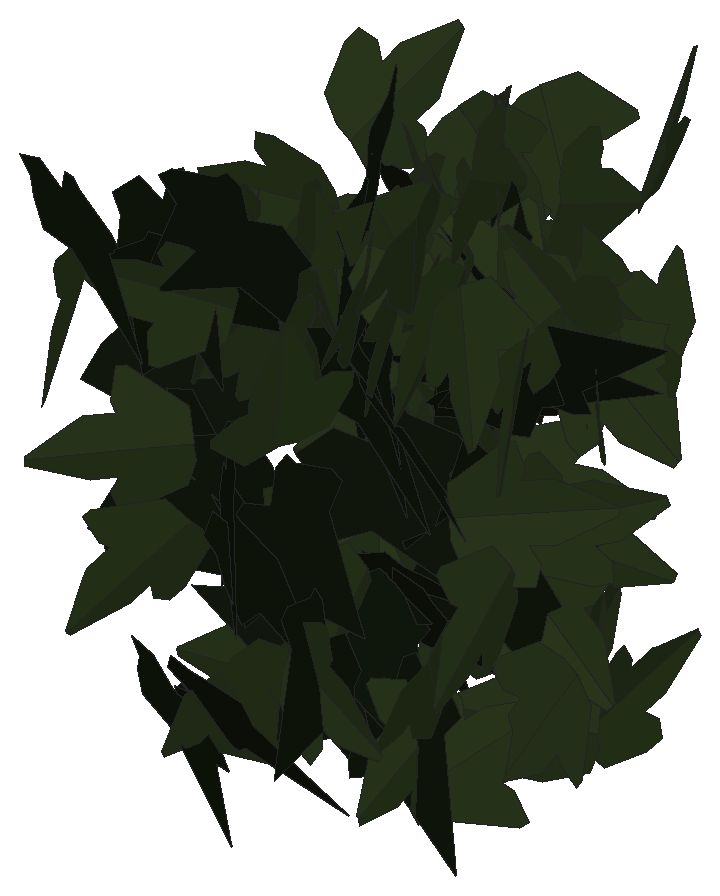
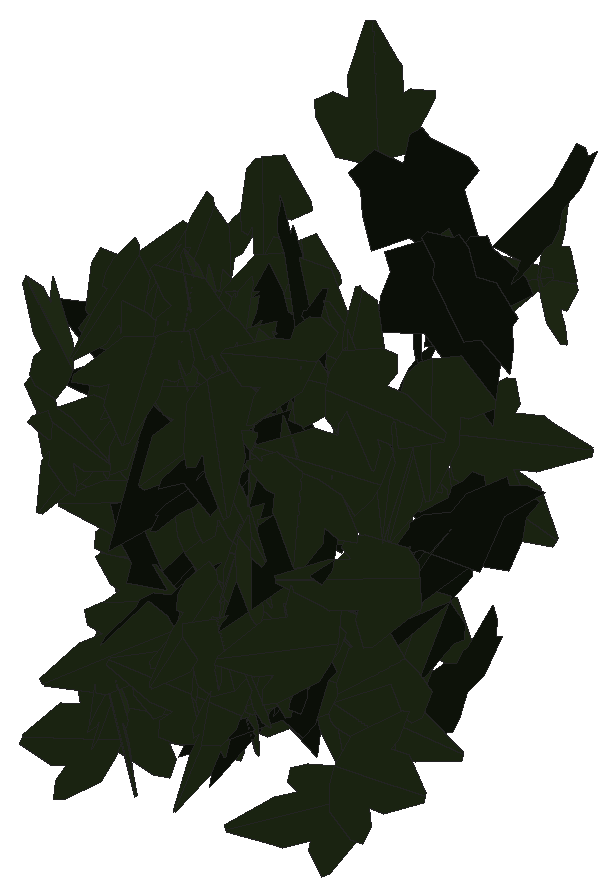
# SketchUp Ruby script. Lengths in inches.
U = 1.inch
M = Sketchup.active_model
def pt(a) = Geom::Point3d.new(a.map { |v| v * U })
def face(e, loops, mat)
  f = e.add_face(loops[0].map { |a| pt(a) })
  loops[1..].each { |l| e.add_face(l.map { |a| pt(a) }).erase! }
  f.material = f.back_material = mat if mat
  f
end
# faces: each face lists its corners as indices into pts; further lists are holes
def faces(e, pts, list, mat = nil) = list.each { |f| face(e, (f[0].is_a?(Array) ? f : [f]).map { |l| l.map { |i| pts[i] } }, mat) }
# xy, xz, yz: faces in a plane at the given z, y or x. An outline is a flat list of corners, or four numbers for a rectangle; further outlines are holes
def ring(l) = l.size == 4 ? [[l[0], l[1]], [l[2], l[1]], [l[2], l[3]], [l[0], l[3]]] : l.each_slice(2).to_a
def flat(e, list, mat, &to3) = list.each { |f| face(e, (f[0].is_a?(Array) ? f : [f]).map { |l| ring(l).map { |u, v| to3.(u, v) } }, mat) }
def xy(e, z, list, mat = nil) = flat(e, list, mat) { |x, y| [x, y, z] }
def xz(e, y, list, mat = nil) = flat(e, list, mat) { |x, z| [x, y, z] }
def yz(e, x, list, mat = nil) = flat(e, list, mat) { |y, z| [x, y, z] }
def lines(e, pts, list) = list.each { |a, b| e.add_line(pt(pts[a]), pt(pts[b])) }
# prism: a flat outline (further loops are holes) pulled along v
def prism(e, loops, v, mat = nil)
  f = face(e, loops, mat); d = Geom::Vector3d.new(v.map { |x| x * U })
  f.pushpull(f.normal.samedirection?(d) ? d.length : -d.length)
end
def box(e, o, s, mat = nil) = prism(e, [[o, [o[0] + s[0], o[1], o[2]], [o[0] + s[0], o[1] + s[1], o[2]], [o[0], o[1] + s[1], o[2]]]], [0, 0, s[2]], mat)
def at(x, y, z, deg = 0) = Geom::Transformation.translation(pt([x, y, z])) * Geom::Transformation.rotation(ORIGIN, Z_AXIS, deg.degrees)
def axes(o, x, y, z) = Geom::Transformation.new([*x, 0, *y, 0, *z, 0, *pt(o).to_a, 1])
def part(name) = M.definitions.add(name)
# library, detail: a bought-in or finely detailed component or shape, given as its bounding box
def library(name, o, s) = part(name).tap { |d| box(d.entities, o, s) }
def detail(e, o, s) = box(e.add_group.entities, o, s)
def put(e, d, t, mat = nil) = e.add_instance(d, t).tap { |i| i.material = mat if mat }
def group(e, t, mat = nil) = e.add_group.tap { |g| g.transformation = t; g.material = mat if mat }.entities
root = M.entities
M.materials.add("efeu1").color = [18, 25, 13]
M.materials.add("efeu2").color = [43, 57, 29]
c1 = part("ivyleaf_10")
p = [[0,0.5,-0.03],[-0.0625,2.02,-0.43],[-0.19,2.01,-0.46],[-0.54,1.05,-0.29],[-0.52,0.625,-0.18],[-0.83,0.76,-0.28],
  [-1.16,0.64,-0.33],[-1.15,0.33,-0.24],[-0.77,-0.39,0.02],[-0.3,-0.51,0.16],[0.04,-0.48,0.23],[-0.02,2.01,-0.4375],
  [-0.06,2.01,-0.43],[0.04,-0.49,0.23],[0.67,-0.49,0.14],[1.38,0.36,-0.2],[1.375,0.51,-0.24],[0.81,0.65,-0.19],
  [0.62,0.59,-0.15],[0.6,1.09,-0.28],[0.5,1.23,-0.31]]
faces(c1.entities,p,[[0,1,2,3,4,5,6,7,8,9,10],[11,12,0,13,14,15,16,17,18,19,20]],"efeu2")
c2 = part("ivyleaf_9")
p = [[1.54,2.16,1.25],[1.36,2.04,1.19],[-0.21,0.99,0.68],[-0.71,1.11,0.82],[-0.85,0.86,0.67],[-0.8,0.17,0.21],
  [-0.9,-0.01,0.1],[-0.67,-0.16,-0.02],[-0.08,-0.08,-0.05],[-0.03,-0.6,-0.4],[0.65,-0.88,-0.66],[0.83,-0.6,-0.49],
  [1.29,-0.42,-0.43],[1.8125,-0.07,-0.26],[1.21,0.44,0.15]]
faces(c2.entities,p,[[0,1,2,3,4,5,6,7,8,9,10,11,12,13,14]],"efeu1")
put(root,c1,axes([15.76,224.72,205.29],[-0.06283,0.04906,0.49361],[-0.33114,0.3663,-0.07855],[-0.36932,-0.33678,-0.01354]))
put(root,c2,axes([15.47,224.3125,204.75],[-0.14625,-0.47747,-0.02524],[0.00758,0.02408,-0.49936],[0.47807,-0.14645,0.00019]))
put(root,c1,axes([15.59,225.57,202.5625],[-0.03739,-0.25538,0.42823],[0.05297,-0.42904,-0.25124],[0.49578,0.02658,0.05913]))
put(root,c1,axes([15.72,224.28,205.94],[-0.08357,-0.48272,-0.09997],[0.02692,0.09678,-0.48981],[0.49223,-0.08725,0.00982]))
put(root,c1,axes([16.13,224.9375,206],[0.05956,0.01203,-0.49629],[-0.48805,0.09294,-0.05632],[0.0909,0.49114,0.02281]))
put(root,c1,axes([15.86,224.29,205.39],[0.0225,-0.33473,-0.37074],[-0.00859,0.37081,-0.3353],[0.49942,0.02146,0.01094]))
put(root,c1,axes([15.53,225.16,204.41],[0.00781,-0.06414,-0.49581],[0.46045,0.19407,-0.01786],[0.19473,-0.45631,0.0621]))
put(root,c1,axes([16.17,223.08,204.72],[-0.02892,-0.02669,0.49845],[-0.30325,-0.39565,-0.03878],[0.39649,-0.30455,0.0067]))
put(root,c1,axes([16.04,224.69,204.98],[-0.13643,-0.48097,-0.00753],[0.00223,0.00719,-0.49994],[0.48102,-0.13645,0.00019]))
put(root,c1,axes([15.82,222.48,206.24],[0.13321,-0.20511,0.4361],[0.26583,-0.34613,-0.24399],[0.40198,0.29686,0.01684]))
put(root,c2,axes([15.71,222.5,206.99],[0.29313,-0.39372,0.09519],[0.05753,-0.07585,-0.49085],[0.40096,0.29872,0.00083]))
put(root,c2,axes([15.79,224.27,204.2],[0.21036,-0.45026,0.05495],[0.02428,-0.04931,-0.49697],[0.45295,0.21175,0.00112]))
put(root,c2,axes([15.97,223.27,204.2],[0.06582,-0.16806,-0.46629],[-0.11073,0.4535,-0.17909],[0.48312,0.12684,0.02248]))
put(root,c1,axes([15.85,225.52,202.15],[-0.02924,-0.09795,-0.48944],[0.3953,0.29481,-0.08261],[0.30477,-0.39178,0.0602]))
put(root,c1,axes([16.5,224.26,202.28],[-0.01794,-0.00235,0.49967],[-0.47822,-0.14488,-0.01785],[0.14487,-0.47854,0.00295]))
put(root,c2,axes([15.97,223.39,206.58],[-0.18584,-0.06121,-0.46013],[0.43336,0.15472,-0.19561],[0.16633,-0.4715,-0.00445]))
put(root,c1,axes([16.07,225.72,205.41],[0.4797,0.0215,0.13937],[0.13869,0.0175,-0.48006],[-0.02552,0.49923,0.01083]))
put(root,c1,axes([16.15,225.53,203.68],[-0.02079,-0.10534,0.48833],[0.0401,0.48683,0.10672],[-0.49796,0.0436,-0.0118]))
put(root,c1,axes([16.08,225,205.23],[-0.08764,-0.22092,0.4399],[0.152,0.41284,0.23761],[-0.4682,0.17538,-0.00521]))
put(root,c1,axes([16.59,223.06,206.12],[-0.12984,0.02802,-0.48203],[-0.46825,-0.12909,0.11863],[-0.11781,0.48223,0.05977]))
put(root,c1,axes([15.91,224.65,203.18],[0.30613,0.07602,0.38795],[0.37679,0.09236,-0.31543],[-0.11962,0.48548,-0.00073]))
put(root,c1,axes([16.42,222.83,204.08],[-0.11373,-0.31356,0.37249],[-0.13234,-0.3482,-0.33353],[0.46856,-0.17445,-0.00379]))
put(root,c2,axes([16.47,223.09,206.39],[0.20451,0.29275,-0.34996],[-0.22048,-0.27235,-0.35667],[-0.39945,0.3002,0.01769]))
put(root,c2,axes([16.05,223.43,202.33],[0.22091,-0.3855,0.22932],[0.11019,-0.20115,-0.44429],[0.43481,0.24683,-0.00392]))
put(root,c1,axes([16.27,225.52,206.5625],[0.18062,0.15706,-0.43899],[0.18473,0.40814,0.22203],[0.42808,-0.24239,0.08941]))
put(root,c1,axes([16.04,224.67,202.46],[-0.06526,-0.015,0.4955],[0.49403,0.03926,0.06626],[-0.0409,0.49823,0.0097]))
put(root,c1,axes([16.51,224.59,205.26],[0.14733,-0.37725,-0.29321],[-0.0089,0.30462,-0.3964],[0.47772,0.12202,0.08304]))
put(root,c2,axes([16.39,225.22,204.9],[0.49076,0.00696,-0.09543],[-0.09554,0.00754,-0.49073],[-0.00539,0.49989,0.00873]))
put(root,c1,axes([16.92,225.35,204.16],[-0.09164,-0.10191,0.48085],[-0.35318,-0.32654,-0.13652],[0.34186,-0.36467,-0.01214]))
put(root,c1,axes([16.7,226.23,206.24],[-0.00117,-0.49927,-0.02693],[0.0006,0.02692,-0.49927],[0.5,-0.0012,0.00054]))
put(root,c1,axes([16.71,224.1,206.24],[0.08895,-0.35534,-0.34032],[-0.01174,0.34421,-0.36247],[0.49188,0.07247,0.05289]))
put(root,c1,axes([16.79,224.48,202.8],[-0.0375,-0.49823,0.01897],[-0.00181,-0.01889,-0.49964],[0.49859,-0.03754,-0.00038]))
put(root,c1,axes([16.74,223.22,202.75],[-0.17653,-0.40832,-0.22829],[0.11011,0.20088,-0.44443],[0.45466,-0.20718,0.01899]))
put(root,c1,axes([16.52,224.52,206],[-0.16226,0.12848,-0.45515],[0.28535,-0.35715,-0.20254],[-0.37716,-0.32548,0.04257]))
put(root,c1,axes([16.87,225.11,205.64],[0.30259,-0.35449,-0.18104],[-0.11969,0.13585,-0.46607],[0.37962,0.3254,-0.00265]))
put(root,c2,axes([17,224.43,202.51],[-0.11716,-0.45808,-0.16259],[-0.04226,-0.15701,0.47282],[-0.48424,0.12453,-0.00193]))
put(root,c1,axes([16.73,225.0625,203.01],[-0.02487,0.07316,0.49399],[0.14637,-0.47182,0.07724],[0.47745,0.14845,0.00205]))
put(root,c1,axes([16.61,225.01,203.17],[0.17938,0.15112,-0.44157],[0.34288,0.27827,0.23452],[0.31663,-0.38695,-0.0038]))
put(root,c2,axes([17.15,222.89,207.09],[0.08905,0.13143,-0.47413],[-0.37355,-0.29553,-0.15208],[-0.32021,0.3813,0.04556]))
put(root,c1,axes([16.62,224.8125,202.86],[0.17627,0.12899,-0.44977],[0.35177,0.28038,0.21827],[0.30852,-0.39338,0.0081]))
put(root,c1,axes([16.94,225.29,205.92],[0.17758,-0.37267,-0.28211],[-0.04572,0.28649,-0.40723],[0.46516,0.17043,0.06767]))
put(root,c1,axes([16.85,225.46,204.37],[0.12139,-0.38738,0.29189],[0.10185,-0.27383,-0.40576],[0.47423,0.15797,0.01243]))
put(root,c2,axes([17.23,224.46,207.01],[-0.0952,0.02704,-0.49011],[-0.45859,0.17312,0.09862],[0.17503,0.46829,-0.00816]))
put(root,c1,axes([16.93,225.47,206.18],[0.10483,-0.39249,0.29148],[0.06972,-0.28306,-0.40622],[0.48389,0.12581,-0.00462]))
put(root,c1,axes([16.99,225.75,203.59],[0.35154,0.3454,-0.08437],[-0.06164,-0.05764,-0.49283],[-0.35017,0.3569,0.00205]))
put(root,c2,axes([16.88,224.8125,206.11],[0.00108,0.01889,-0.49964],[0.39432,-0.30723,-0.01076],[-0.30742,-0.39402,-0.01556]))
put(root,c2,axes([16.93,225.71,205.56],[-0.05339,-0.47792,-0.13689],[0.02753,0.13463,-0.48075],[0.49638,-0.05887,0.01194]))
put(root,c1,axes([17.36,225.12,206],[-0.16907,0.2419,-0.40361],[-0.29601,0.27871,0.29103],[0.36578,0.33736,0.04897]))
put(root,c2,axes([16.71,222.9,202.78],[0.43197,-0.15711,0.19677],[0.18785,-0.05913,-0.45958],[0.16768,0.47098,0.00794]))
put(root,c2,axes([16.87,224.83,203.04],[0.49315,0.07077,0.04238],[0.04143,0.00963,-0.49819],[-0.07133,0.49487,0.00363]))
put(root,c1,axes([17.53,225.24,204.86],[-0.21982,0.05639,0.44553],[-0.44507,0.03886,-0.22451],[-0.05995,-0.49529,0.03311]))
put(root,c1,axes([17.06,224.29,203.18],[-0.04188,-0.21562,0.44917],[0.23027,-0.4081,-0.17444],[0.44184,0.19225,0.13348]))
put(root,c2,axes([17.11,224.81,203.06],[0.46012,0.03219,-0.193],[-0.19272,-0.01076,-0.46124],[-0.03385,0.49885,0.0025]))
put(root,c1,axes([17.14,225.35,203.07],[0.4045,-0.2858,0.06856],[0.05896,-0.03535,-0.49525],[0.28793,0.40874,0.0051]))
put(root,c1,axes([17.24,225.64,203.78],[-0.02251,-0.21735,-0.44972],[0.06355,0.44528,-0.21838],[0.49543,-0.06699,0.00758]))
put(root,c1,axes([16.86,224.8,205.85],[0.02973,-0.08047,-0.49259],[0.49907,0.01113,0.02831],[0.00641,-0.49336,0.08098]))
put(root,c2,axes([17.11,224.36,203],[0.16156,-0.40572,-0.2435],[-0.07677,0.23141,-0.43652],[0.46691,0.17844,0.01248]))
put(root,c1,axes([17.28,225.4,202.58],[0.06832,-0.35484,-0.34557],[0.08286,0.35212,-0.34518],[0.48833,-0.01011,0.10692]))
put(root,c1,axes([16.92,225.11,203.52],[0.04863,-0.00425,-0.49761],[0.4681,-0.16929,0.04719],[-0.16888,-0.47045,-0.01249]))
put(root,c1,axes([17.54,225.23,203.29],[0.04692,-0.03461,-0.49659],[-0.25361,0.42754,-0.05376],[0.42835,0.25692,0.02256]))
put(root,c1,axes([17.41,224.7,204.18],[0.07243,-0.16283,-0.46716],[-0.03967,0.46871,-0.16952],[0.49313,0.06162,0.05498]))
put(root,c1,axes([17.31,224.41,206.51],[-0.33489,-0.32478,-0.1799],[0.13167,0.12262,-0.4665],[0.34714,-0.35983,0.0034]))
put(root,c1,axes([17.34,224.85,205.9375],[0.07859,-0.11078,-0.4812],[0.05341,0.4863,-0.10323],[0.49089,-0.03518,0.08827]))
put(root,c1,axes([17.11,225.61,205.68],[0.23736,0.24847,0.36322],[0.24673,0.26658,-0.3436],[-0.3644,0.34234,0.00394]))
put(root,c1,axes([17.67,225.13,204.1],[-0.35851,0.06508,-0.34239],[-0.33996,0.0429,0.36412],[0.07677,0.49389,0.01349]))
put(root,c2,axes([17.31,223.0625,204.54],[0.15084,-0.26384,-0.39704],[-0.19323,0.34685,-0.3039],[0.43579,0.24512,0.00267]))
put(root,c2,axes([17.1,224.45,205.29],[-0.05207,-0.03915,-0.49574],[0.49702,-0.02019,-0.05061],[-0.01605,-0.49806,0.04102]))
put(root,c1,axes([17.4,224.94,205.84],[0.21186,-0.44519,0.08319],[0.04733,-0.06958,-0.49287],[0.45042,0.21671,0.01266]))
put(root,c2,axes([17.05,225.11,206.09],[0.22101,-0.21708,0.39247],[0.27075,-0.28424,-0.30968],[0.35756,0.3494,-0.00809]))
put(root,c2,axes([17.36,225.67,204.97],[-0.10432,-0.44662,0.19911],[-0.01779,-0.19999,-0.45792],[0.48867,-0.10263,0.02583]))
put(root,c1,axes([17.15,225.65,202.79],[-0.13577,-0.1145,0.46739],[0.36414,0.29304,0.17757],[-0.31459,0.38861,0.00381]))
put(root,c1,axes([17.4,226.3,206.59],[0.18481,0.45724,0.08234],[0.03008,0.07666,-0.49317],[-0.46362,0.18724,0.00083]))
put(root,c1,axes([17.57,223.77,206.31],[0.16964,-0.44657,-0.14765],[-0.04307,0.14155,-0.47761],[0.46837,0.17476,0.00956]))
put(root,c2,axes([17.24,222.57,204.99],[-0.01282,-0.08673,-0.49225],[0.48526,-0.12022,0.00855],[-0.11984,-0.47752,0.08725]))
put(root,c1,axes([17.22,225.37,206.18],[0.30308,-0.11246,0.38144],[0.36737,-0.10445,-0.32269],[0.15226,0.47586,0.01932]))
put(root,c2,axes([17.28,224.32,204.52],[-0.10264,-0.17983,-0.45511],[0.27759,0.36156,-0.20547],[0.403,-0.29485,0.02562]))
put(root,c1,axes([17.4,224.4,205.82],[0.15761,0.16125,-0.44627],[0.24389,0.37585,0.22194],[0.40703,-0.28764,0.03983]))
put(root,c1,axes([17.25,225.5625,206.69],[0.34887,0.07018,0.35123],[0.33119,0.1235,-0.35364],[-0.13639,0.4794,0.03969]))
put(root,c2,axes([17.29,224,205.42],[0.30821,-0.39086,0.04726],[0.02615,-0.03956,-0.49775],[0.39284,0.30929,-0.00395]))
put(root,c2,axes([17.38,222.53,204.6],[0.35293,-0.30645,-0.17758],[-0.12165,0.13056,-0.46707],[0.33263,0.37289,0.0176]))
put(root,c1,axes([17.52,225.24,206.28],[0.24684,-0.42501,0.09185],[-0.04367,0.08085,0.49148],[-0.43263,-0.25065,0.00279]))
put(root,c1,axes([17.25,225.27,205.71],[0.07463,-0.03824,-0.49292],[0.49245,-0.03842,0.07754],[-0.0438,-0.49705,0.03193]))
put(root,c1,axes([17.4375,225.71,206.43],[-0.03895,0.04067,0.49682],[0.36988,-0.33171,0.05616],[0.33417,0.37191,-0.00424]))
put(root,c1,axes([17.42,225.08,206.11],[-0.1971,0.05509,0.4562],[0.40116,-0.22146,0.20006],[0.2241,0.44488,0.0431]))
put(root,c1,axes([17.97,224.92,205.96],[0.25694,0.20482,0.37687],[-0.31401,-0.20945,0.32792],[0.2922,-0.40519,0.021]))
put(root,c2,axes([18.05,224.87,203.61],[0.07577,0.07071,-0.48914],[-0.3935,-0.29078,-0.10299],[-0.29903,0.40056,0.01159]))
put(root,c2,axes([17.5,224.3,202.46],[-0.17242,-0.09555,-0.4595],[0.43255,0.15761,-0.19508],[0.18212,-0.46479,0.02831]))
put(root,c2,axes([18.14,224.875,206.1],[-0.21041,0.00753,-0.45351],[-0.45297,0.02234,0.21053],[0.02343,0.49944,-0.00258]))
put(root,c1,axes([17.75,224.03,206.21],[0.21532,-0.42797,0.1431],[0.06878,-0.12558,-0.47906],[0.44599,0.22599,0.0048]))
put(root,c1,axes([17.45,225.66,202.84],[0.00696,-0.01252,0.49979],[0.4873,-0.11155,-0.00958],[0.11174,0.48724,0.01065]))
put(root,c1,axes([17.75,224.33,202.18],[-0.13991,-0.11313,0.46651],[0.17149,-0.46563,-0.06149],[0.44835,0.1428,0.16909]))
put(root,c1,axes([17.8,224.55,205.94],[0.08034,-0.37493,0.3209],[0.11148,-0.30293,-0.38185],[0.48075,0.1329,0.03493]))
put(root,c2,axes([17.74,225.55,203.625],[0.02926,-0.46907,-0.17062],[-0.00834,0.17043,-0.46998],[0.49907,0.03035,0.00215]))
put(root,c1,axes([17.96,224.72,206.97],[0.02275,-0.27045,-0.41993],[0.00328,0.42043,-0.2706],[0.49947,0.00955,0.0209]))
put(root,c2,axes([17.86,224.9,205.0625],[0.2767,0.38347,0.16244],[0.09349,0.13285,-0.47287],[-0.40583,0.29206,0.00182]))
put(root,c2,axes([17.68,224.1,204.95],[0.18303,-0.32182,0.33605],[0.20622,-0.26761,-0.36859],[0.4171,0.27353,0.03477]))
put(root,c1,axes([18.1,223.73,206.95],[0.04458,-0.46715,-0.17258],[-0.01872,0.17158,-0.46927],[0.49766,0.0483,-0.00219]))
put(root,c1,axes([17.77,225.85,203.29],[-0.18774,-0.11577,-0.44872],[0.40328,0.1977,-0.21974],[0.2283,-0.44442,0.01914]))
put(root,c2,axes([18.02,224.88,203.64],[0.34868,0.16825,0.31641],[-0.29608,-0.11347,0.3866],[0.20189,-0.45697,0.0205]))
put(root,c1,axes([18.4,225.27,202.09],[0.01964,0.0169,0.49933],[-0.41747,-0.27396,0.0257],[0.27447,-0.41792,0.00335]))
put(root,c1,axes([18.13,223.91,203.05],[-0.00126,-0.43706,-0.24285],[-0.00433,0.24285,-0.43704],[0.49998,0.001,-0.00439]))
put(root,c1,axes([18.24,225.77,202.66],[0.26003,-0.35717,-0.23412],[-0.14214,0.1861,-0.44177],[0.40272,0.2963,-0.00475]))
put(root,c2,axes([17.96,222.87,203.69],[0.11175,-0.0914,-0.4787],[0.35991,-0.31566,0.14429],[-0.32859,-0.37684,-0.00476]))
put(root,c1,axes([18.4375,225.54,202.58],[0.01619,-0.03777,0.49831],[-0.31965,0.38246,0.03937],[-0.38414,-0.31984,-0.01176]))
put(root,c1,axes([18.13,225.48,206.07],[-0.44422,0.06052,-0.22137],[0.21843,-0.03643,-0.44829],[-0.07039,-0.49499,0.00593]))
put(root,c1,axes([17.97,224.35,201.96],[0.28663,0.08513,-0.40075],[0.38469,0.11231,0.299],[0.14092,-0.47973,-0.00112]))
put(root,c1,axes([17.94,222.62,203.52],[0.09,-0.02698,0.49109],[0.49107,-0.0228,-0.09125],[0.02732,0.49875,0.02239]))
put(root,c2,axes([17.98,224.67,205.35],[0.15979,0.21142,-0.42399],[0.25801,0.33645,0.26501],[0.39736,-0.30348,-0.00157]))
put(root,c1,axes([18.3125,226.46,206.36],[0.24622,-0.40706,0.15389],[-0.06403,0.141,0.47542],[-0.43044,-0.25382,0.0173]))
put(root,c1,axes([18.38,225.35,206.625],[0.05347,-0.21893,-0.44633],[0.07705,0.44713,-0.21009],[0.49112,-0.04632,0.08156]))
put(root,c1,axes([18.79,226.02,205.25],[0.083,0.08005,0.48652],[-0.4911,0.05744,0.07433],[-0.04399,-0.4902,0.08816]))
put(root,c1,axes([18.47,225.7,201.98],[0.05922,-0.21247,0.44872],[-0.05155,0.44683,0.21837],[-0.4938,-0.07213,0.03102]))
put(root,c1,axes([18.2,225.08,203.22],[0.31727,0.1479,0.35703],[0.3249,0.14804,-0.35004],[-0.20925,0.4541,-0.00216]))
put(root,c1,axes([18.17,225.0625,204.24],[-0.085,-0.03935,-0.49115],[0.48312,0.09127,-0.09092],[0.09681,-0.49002,0.0225]))
put(root,c1,axes([18.71,224.9,205.9],[-0.41325,-0.14873,-0.23896],[-0.21558,-0.10567,0.43859],[-0.18097,0.46552,0.02321]))
put(root,c1,axes([18.51,223.9,206.27],[0.02966,0.49549,-0.06006],[-0.00775,-0.0597,-0.49636],[-0.49906,0.03038,0.00414]))
put(root,c1,axes([18.6,224.86,205.98],[-0.0841,-0.09082,0.48444],[0.08269,-0.48707,-0.07696],[0.48589,0.06717,0.09694]))
put(root,c2,axes([18.2,224.8,205.42],[0.14619,-0.10485,0.46651],[0.46365,-0.08814,-0.16511],[0.11686,0.48087,0.07146]))
put(root,c1,axes([18.59,221.5625,206.4],[-0.16203,-0.46665,-0.07737],[-0.02376,-0.07365,0.49397],[-0.47242,0.16375,0.0017]))
put(root,c1,axes([18.5,225.41,204.86],[-0.36446,0.18111,0.29046],[0.25516,-0.13907,0.40688],[0.22817,0.44481,0.00894]))
put(root,c1,axes([18.43,224.22,204.36],[-0.029,-0.01795,0.49884],[0.26947,0.42005,0.03077],[-0.42017,0.27063,-0.01469]))
put(root,c1,axes([18.53,225.54,205.125],[0.15249,0.38226,0.28394],[0.10259,0.26477,-0.41155],[-0.465,0.18378,0.00231]))
put(root,c1,axes([18.63,224.06,203.83],[-0.017,-0.26816,0.42167],[0.16459,-0.40137,-0.24862],[0.47183,0.13035,0.10192]))
put(root,c1,axes([18.42,224.96,203.97],[-0.15032,-0.13118,0.45847],[0.3565,0.28835,0.19939],[-0.31672,0.38684,0.00684]))
put(root,c1,axes([18.58,224.43,205.7],[0.30871,-0.30713,0.24569],[0.18459,-0.16266,-0.43528],[0.34731,0.35946,0.01296]))
put(root,c1,axes([18.84,224.58,202.81],[0.42483,-0.15663,-0.2121],[-0.19734,0.07787,-0.45276],[0.17486,0.46841,0.00434]))
